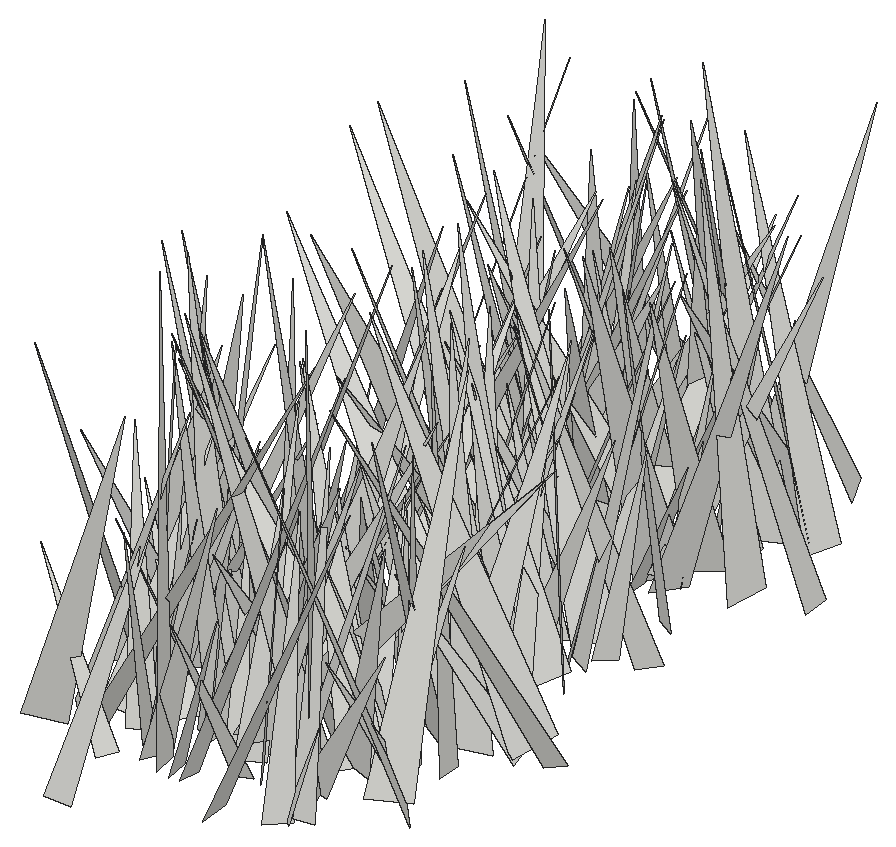
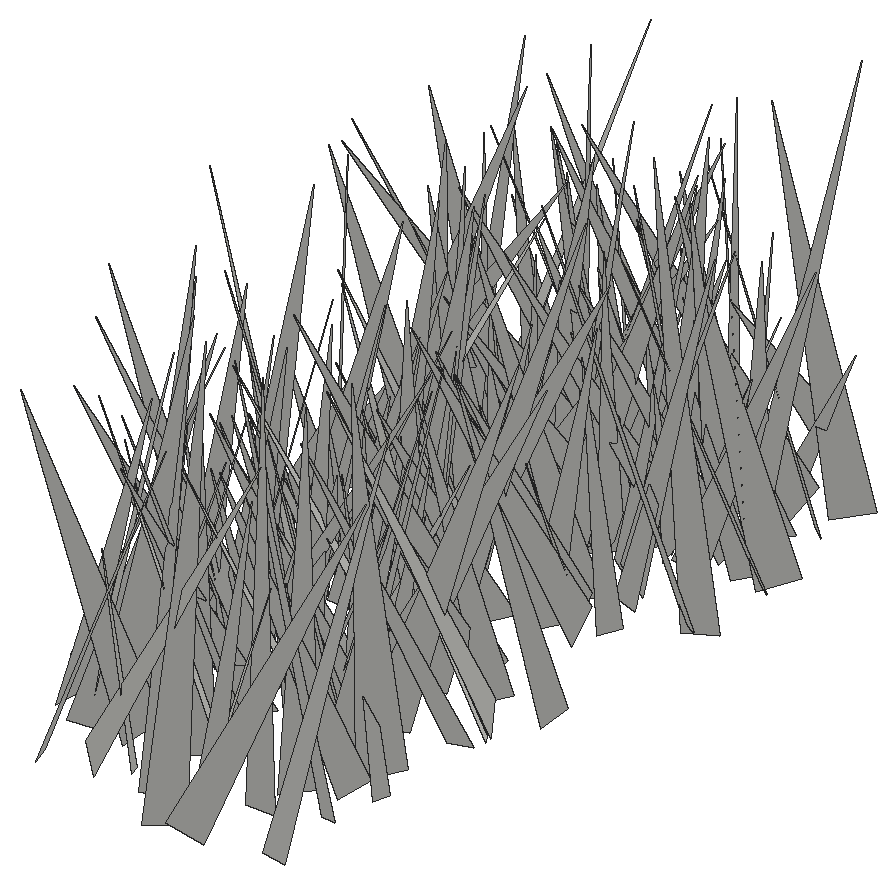
# SketchUp Ruby script. Lengths in inches.
U = 1.inch
M = Sketchup.active_model
def pt(a) = Geom::Point3d.new(a.map { |v| v * U })
def face(e, loops, mat)
  f = e.add_face(loops[0].map { |a| pt(a) })
  loops[1..].each { |l| e.add_face(l.map { |a| pt(a) }).erase! }
  f.material = f.back_material = mat if mat
  f
end
# faces: each face lists its corners as indices into pts; further lists are holes
def faces(e, pts, list, mat = nil) = list.each { |f| face(e, (f[0].is_a?(Array) ? f : [f]).map { |l| l.map { |i| pts[i] } }, mat) }
# xy, xz, yz: faces in a plane at the given z, y or x. An outline is a flat list of corners, or four numbers for a rectangle; further outlines are holes
def ring(l) = l.size == 4 ? [[l[0], l[1]], [l[2], l[1]], [l[2], l[3]], [l[0], l[3]]] : l.each_slice(2).to_a
def flat(e, list, mat, &to3) = list.each { |f| face(e, (f[0].is_a?(Array) ? f : [f]).map { |l| ring(l).map { |u, v| to3.(u, v) } }, mat) }
def xy(e, z, list, mat = nil) = flat(e, list, mat) { |x, y| [x, y, z] }
def xz(e, y, list, mat = nil) = flat(e, list, mat) { |x, z| [x, y, z] }
def yz(e, x, list, mat = nil) = flat(e, list, mat) { |y, z| [x, y, z] }
def lines(e, pts, list) = list.each { |a, b| e.add_line(pt(pts[a]), pt(pts[b])) }
# prism: a flat outline (further loops are holes) pulled along v
def prism(e, loops, v, mat = nil)
  f = face(e, loops, mat); d = Geom::Vector3d.new(v.map { |x| x * U })
  f.pushpull(f.normal.samedirection?(d) ? d.length : -d.length)
end
def box(e, o, s, mat = nil) = prism(e, [[o, [o[0] + s[0], o[1], o[2]], [o[0] + s[0], o[1] + s[1], o[2]], [o[0], o[1] + s[1], o[2]]]], [0, 0, s[2]], mat)
def at(x, y, z, deg = 0) = Geom::Transformation.translation(pt([x, y, z])) * Geom::Transformation.rotation(ORIGIN, Z_AXIS, deg.degrees)
def axes(o, x, y, z) = Geom::Transformation.new([*x, 0, *y, 0, *z, 0, *pt(o).to_a, 1])
def part(name) = M.definitions.add(name)
# library, detail: a bought-in or finely detailed component or shape, given as its bounding box
def library(name, o, s) = part(name).tap { |d| box(d.entities, o, s) }
def detail(e, o, s) = box(e.add_group.entities, o, s)
def put(e, d, t, mat = nil) = e.add_instance(d, t).tap { |i| i.material = mat if mat }
def group(e, t, mat = nil) = e.add_group.tap { |g| g.transformation = t; g.material = mat if mat }.entities
root = M.entities
c1 = part("fur_instance\#9")
p = [[0.8125,0,1.79],[0.67,-0.02,1.48],[0,-0.11,0],[0,0.11,0]]
faces(c1.entities,p,[[0,1,2,3]])
put(root,c1,axes([470.51,80.25,-21.66],[-3.32037,-5.8988,2.51801],[-6.36421,2.67847,-2.11746],[-0.7956,3.19234,6.42939]))
put(root,c1,axes([468.38,101.12,-21.86],[-2.99336,-6.46525,0.18966],[-6.30073,2.9619,1.52434],[1.46161,-0.47255,6.9596]))
put(root,c1,axes([470.64,92.61,-21.66],[-5.74656,4.30747,2.03787],[4.75581,5.38477,2.02895],[0.29923,-2.86007,6.88916]))
put(root,c1,axes([469.65,78.47,-21.66],[1.26749,-5.25605,0.55346],[-5.00773,-1.37633,-1.60227],[-1.68968,0.13629,5.16385]))
put(root,c1,axes([467.07,88.49,-21.86],[6.15775,0.09619,0.89999],[0.03195,-6.20791,0.44493],[-0.90455,0.43558,6.14241]))
put(root,c1,axes([469.07,94.78,-21.86],[-5.99811,4.4385,2.51735],[4.45899,6.44808,-0.74453],[2.48087,-0.8583,7.4245]))
put(root,c1,axes([470.49,72.26,-21.86],[-1.80359,3.13263,0.44398],[3.00697,1.53819,1.36218],[-0.98418,-1.04117,3.34825]))
put(root,c1,axes([468.84,76.53,-21.86],[-3.41876,-7.6362,0.72671],[-7.48826,3.49493,1.49637],[1.66304,0.03883,8.23167]))
put(root,c1,axes([466.91,77.29,-21.86],[5.22316,-4.20753,1.34718],[-4.41725,-5.01042,1.47756],[-0.07792,1.998,6.54228]))
put(root,c1,axes([466.87,81.31,-21.86],[0.15208,-7.64456,1.76209],[-7.47072,0.39677,2.36609],[2.3943,1.72356,7.27077]))
put(root,c1,axes([468.41,89.93,-21.66],[6.47169,4.71895,0.84374],[4.29058,-6.33416,2.51645],[-2.13805,1.57262,7.60387]))
put(root,c1,axes([467.27,77.71,-21.86],[3.93505,4.96293,0.50565],[4.97977,-3.8695,-0.7745],[0.29702,-0.87596,6.28613]))
put(root,c1,axes([469.98,81.29,-21.86],[-1.24841,-4.57565,0.91997],[-4.66472,1.19209,-0.401],[-0.15278,0.99186,4.72592]))
put(root,c1,axes([472.93,89.31,-21.86],[-4.85114,5.94494,0.47809],[5.69058,4.42924,2.66526],[-1.78556,-2.03568,7.19529]))
put(root,c1,axes([471.02,75.84,-21.86],[-2.26305,3.25436,0.20739],[3.19812,2.16563,0.91504],[-0.63708,-0.68879,3.8568]))
put(root,c1,axes([473.08,76.92,-21.86],[-7.866,-1.33504,0.19154],[-1.32695,7.45779,-2.51268],[-0.24134,2.50839,7.5725]))
put(root,c1,axes([468.86,74.78,-21.86],[-1.32926,4.80497,0.97182],[4.66035,1.55098,-1.29408],[1.52094,-0.553,4.81456]))
put(root,c1,axes([470.34,74.24,-21.86],[-1.55203,4.86816,1.43833],[5.0761,1.479,0.47157],[-0.03172,-1.51332,5.08777]))
put(root,c1,axes([467.65,72.6,-21.66],[4.01839,-5.64573,1.18023],[-5.73753,-3.76564,1.52164],[0.58986,1.83314,6.76065]))
put(root,c1,axes([470.63,75.46,-21.86],[-7.01527,0.64484,2.20419],[0.06996,7.14138,-1.86657],[2.29551,1.75305,6.79307]))
put(root,c1,axes([470.91,77.6875,-21.86],[-4.6642,0.46344,0.8289],[0.1067,4.38406,-1.85075],[0.94364,1.79496,4.30631]))
put(root,c1,axes([471.59,101.64,-21.86],[1.60402,-6.13136,0.73735],[-5.58582,-1.76536,-2.52831],[-2.63361,0.00991,5.81155]))
put(root,c1,axes([468.12,95.96,-21.86],[5.21952,0.68023,0.61562],[0.83808,-4.98198,-1.60081],[-0.37326,-1.674,5.01433]))
put(root,c1,axes([467.94,90.85,-21.86],[3.62695,2.69385,0.06353],[2.59465,-3.4627,-1.30122],[0.7271,-1.08099,4.32648]))
put(root,c1,axes([467.18,81.49,-21.66],[5.13352,5.29295,1.04527],[5.31008,-4.70157,-2.27141],[0.95446,-2.31104,7.01492]))
put(root,c1,axes([468.11,73.8125,-21.86],[4.67492,4.49227,1.13099],[4.6277,-4.45606,-1.42912],[0.20972,-1.8104,6.324]))
put(root,c1,axes([468.34,91.6875,-21.86],[1.18506,6.07091,0.5983],[5.8889,-0.9794,-1.72625],[1.5921,-0.89616,5.93973]))
put(root,c1,axes([469.21,82.99,-21.86],[4.35751,-1.25814,0.68683],[-1.21703,-4.4086,-0.35441],[-0.75729,-0.15444,4.52164]))
put(root,c1,axes([473.0625,91.98,-21.66],[-7.26619,-2.16018,0.91047],[-2.32448,7.02333,-1.88745],[0.30351,2.07347,7.34176]))
put(root,c1,axes([471.36,76.4375,-21.86],[-2.85386,-2.94003,0.13695],[-2.93623,2.85714,0.14971],[0.2028,-0.00613,4.09462]))
put(root,c1,axes([471.38,77.2,-21.86],[-7.46216,1.5868,2.36089],[1.65538,7.81249,-0.01867],[2.31332,-0.47194,7.62898]))
put(root,c1,axes([471.58,93.05,-21.86],[-6.2182,-2.45212,1.53392],[-2.39925,6.40419,0.51167],[1.61537,0.0727,6.66461]))
put(root,c1,axes([471.03,82.51,-21.66],[1.74005,3.73475,0.21366],[3.48509,-1.70407,1.40429],[-1.35946,0.41179,3.87351]))
put(root,c1,axes([470.57,95.25,-21.86],[3.73723,-3.51523,0.8829],[-3.22394,-3.80362,-1.49732],[-1.65607,-0.52811,4.90732]))
put(root,c1,axes([471.1,68.95,-21.86],[-4.90566,2.32822,0.51514],[1.6552,4.17303,-3.098],[1.71648,2.62995,4.45965]))
put(root,c1,axes([470.23,87.96,-21.86],[5.42222,1.22065,1.50489],[0.3801,-5.05507,2.73075],[-1.90005,2.47215,4.84081]))
put(root,c1,axes([468.04,77.6,-21.86],[0.54416,-5.67013,1.84078],[-5.27926,0.40028,2.79359],[2.76917,1.87733,4.9641]))
put(root,c1,axes([470.67,74.41,-21.86],[-4.89725,-3.9807,3.26033],[-4.56553,5.43754,-0.21877],[2.37312,2.24631,6.30723]))
put(root,c1,axes([470.1,83.29,-21.86],[7.02675,2.35333,1.41841],[1.60681,-6.67867,3.12071],[-2.22895,2.60433,6.72121]))
put(root,c1,axes([471.99,75.27,-21.86],[4.59054,6.55576,1.84003],[6.00661,-4.94402,2.62946],[-3.20693,0.124,7.5589]))
put(root,c1,axes([471.59,89.53,-21.86],[6.1806,-4.85252,1.92283],[-3.89661,-6.27237,-3.30423],[-3.47285,-1.59827,7.12944]))
put(root,c1,axes([471.51,79.5625,-21.86],[-3.91198,-5.41617,1.52932],[-5.50053,4.07361,0.35664],[1.19076,1.02376,6.67167]))
put(root,c1,axes([470.56,74.21,-21.86],[2.84043,2.51238,0.82611],[2.52394,-2.93724,0.2547],[-0.79009,-0.35083,3.78354]))
put(root,c1,axes([468.93,96.34,-21.66],[5.6454,-1.61471,0.55375],[-1.70236,-5.46688,1.41409],[-0.12614,1.5134,5.69896]))
put(root,c1,axes([470.64,74.18,-21.86],[4.23217,0.79223,1.75299],[1.35483,-4.23497,-1.35698],[-1.36567,-1.74623,4.08626]))
put(root,c1,axes([468.37,98.36,-21.66],[5.01746,5.30698,2.27397],[5.71554,-4.13917,-2.95123],[0.81705,-3.63499,6.68051]))
put(root,c1,axes([470.44,97.27,-21.86],[5.51508,-3.1001,1.56666],[-3.03836,-5.73026,-0.64316],[-1.68328,0.18611,6.29389]))
put(root,c1,axes([469.2,76.88,-21.66],[5.44463,0.12063,0.24069],[0.04962,-5.23956,1.50366],[-0.26462,1.49964,5.23426]))
put(root,c1,axes([470.77,82.32,-21.86],[5.48783,2.36239,1.1528],[1.72376,-5.24883,2.55038],[-1.98455,1.97355,5.40302]))
put(root,c1,axes([472.52,72.66,-21.66],[-7.45834,-2.27512,2.73301],[-2.96816,7.48025,-1.87304],[1.95846,2.67246,7.56933]))
put(root,c1,axes([472.49,75.58,-21.86],[-6.61174,-0.50833,1.66504],[-0.62205,6.79727,-0.39495],[1.62598,0.53342,6.61948]))
put(root,c1,axes([470.8125,83.7,-21.86],[-3.2571,5.60614,0.8435],[5.30317,3.35677,-1.83235],[2.00417,0.22864,6.21933]))
put(root,c1,axes([469.28,88.66,-21.86],[3.19208,-3.97574,0.46961],[-3.91795,-2.97897,1.41133],[0.82265,1.2392,4.89939]))
put(root,c1,axes([472.45,78.92,-21.66],[-6.55431,0.09701,1.7896],[-0.34688,6.588,-1.62754],[1.75834,1.66126,6.34976]))
put(root,c1,axes([472.17,82.44,-21.86],[-0.83956,4.61048,2.28414],[5.1209,0.52371,0.82514],[-0.50027,-2.37653,4.61309]))
put(root,c1,axes([472.4,95.2,-21.86],[-4.41173,-1.92667,0.46008],[-1.77307,4.34177,1.17998],[0.88316,-0.90777,4.66723]))
put(root,c1,axes([470.45,99.21,-21.66],[-1.45623,-6.82166,1.9418],[-6.84757,1.86878,1.42991],[1.84835,1.54881,6.82723]))
put(root,c1,axes([469.75,76.44,-21.86],[3.43659,4.37627,1.35344],[4.55407,-3.08156,-1.59944],[0.49399,-2.03617,5.32951]))
put(root,c1,axes([475.37,83.7,-21.86],[-5.71693,5.39586,0.3581],[5.20349,5.34707,2.50186],[-1.47216,-2.05434,7.45247]))
put(root,c1,axes([472.47,91.63,-21.86],[-5.1029,2.41175,1.4356],[2.37658,5.2976,-0.4521],[1.4931,-0.1897,5.62599]))
put(root,c1,axes([472.86,98.9375,-21.86],[-3.26871,-2.2439,0.63682],[-2.29753,3.28654,-0.21245],[0.40248,0.53729,3.95909]))
put(root,c1,axes([471.55,76.61,-21.86],[6.78257,3.66457,1.14232],[2.83952,-6.35069,3.51329],[-2.58286,2.6414,6.86216]))
put(root,c1,axes([473.46,80.1,-21.66],[-0.04463,-6.97717,1.39975],[-6.92736,-0.27772,-1.60522],[-1.62845,1.37265,6.79015]))
put(root,c1,axes([471.07,94.03,-21.86],[3.65147,4.43575,1.22236],[4.5601,-3.69672,-0.20725],[-0.61278,-1.07778,5.74161]))
put(root,c1,axes([472.53,99.3,-21.86],[-1.33118,-5.02308,1.66852],[-5.29255,1.28443,-0.35575],[0.06525,1.70478,5.18429]))
put(root,c1,axes([472.21,82.57,-21.66],[-4.0426,1.99311,1.15136],[1.52694,4.06338,-1.67276],[1.72237,1.07573,4.18533]))
put(root,c1,axes([471.67,94.47,-21.66],[4.6203,4.92142,0.32663],[4.69042,-4.52255,1.79463],[-1.52544,1.00021,6.50745]))
put(root,c1,axes([469.33,72.95,-21.66],[7.73901,0.54751,0.09462],[0.50511,-7.48314,1.98706],[-0.23147,1.9758,7.49957]))
put(root,c1,axes([473,89.42,-21.86],[-0.62514,-3.66803,1.11265],[-3.82799,0.53943,-0.37244],[-0.19721,1.15663,3.70223]))
put(root,c1,axes([470.14,87.85,-21.66],[7.35163,-0.33714,0.71191],[-0.54127,-7.01692,2.26646],[-0.57229,2.30568,7.00167]))
put(root,c1,axes([472.29,84.82,-21.66],[-2.9389,4.8588,0.20427],[4.55933,2.83593,-1.85926],[1.6918,0.79774,5.36547]))
put(root,c1,axes([474.28,89.21,-21.86],[-2.77092,-3.22119,0.17285],[-3.17409,2.68192,-0.90354],[-0.57541,0.71776,4.15182]))
put(root,c1,axes([473.98,79.47,-21.86],[-7.67624,-2.38765,2.18106],[-2.53698,7.93,-0.24775],[2.0054,0.89261,8.03519]))
put(root,c1,axes([473.28,75.37,-21.86],[-0.33834,3.74046,0.53618],[3.75079,0.26714,0.50319],[-0.45836,-0.57497,3.72187]))
put(root,c1,axes([474.47,87.67,-21.66],[0.43766,-5.35462,0.13989],[-4.92597,-0.45748,-2.09965],[-2.10387,-0.04276,4.94519]))
put(root,c1,axes([472.75,79.39,-21.86],[3.27584,-2.78093,0.2499],[-2.38988,-2.99185,-1.96583],[-1.44378,-1.35736,3.82103]))
put(root,c1,axes([471.39,76.43,-21.86],[3.86855,-0.79855,0.19754],[-0.81455,-3.85123,0.38332],[-0.11496,0.41562,3.93147]))
put(root,c1,axes([472,95.17,-21.86],[5.42096,2.25752,1.64956],[2.38588,-5.61122,-0.16143],[-1.45775,-0.7887,5.87002]))
put(root,c1,axes([476.5,78.19,-21.66],[-6.39943,2.86094,0.01202],[2.71801,6.07041,2.2137],[-0.89308,-2.0256,6.65111]))
put(root,c1,axes([473.33,93.72,-21.86],[0.82489,5.68831,1.342],[5.81529,-0.93413,0.38496],[-0.58339,-1.2684,5.73491]))
put(root,c1,axes([471.18,81.78,-21.86],[2.35297,-5.60644,2.50548],[-6.03434,-1.6135,2.05656],[1.13856,3.03489,5.72182]))
put(root,c1,axes([471.32,92.89,-21.66],[6.28882,0.29269,0.74734],[0.08478,-6.11246,1.68051],[-0.79813,1.65699,6.06719]))
put(root,c1,axes([471.73,73.21,-21.86],[5.0608,-1.8582,0.79428],[-1.91101,-5.09708,0.2516],[-0.65714,0.51221,5.38529]))
put(root,c1,axes([475.91,77.33,-21.66],[-4.08084,-6.31933,0.93728],[-6.28934,3.77891,-1.90517],[-1.12095,1.80323,7.27719]))
put(root,c1,axes([472,81.39,-21.86],[4.40688,2.08061,0.00975],[2.02682,-4.29803,1.08102],[-0.47012,0.97349,4.75194]))
put(root,c1,axes([476.33,93.375,-21.86],[-7.00038,0.48524,0.02911],[0.47648,6.76613,1.79834],[-0.09628,-1.796,6.78283]))
put(root,c1,axes([475.12,93.96,-21.86],[-4.76571,-0.2474,0.30777],[-0.30187,4.68534,-0.90794],[0.25457,0.92426,4.68496]))
put(root,c1,axes([470.7,94.47,-21.66],[2.62599,-5.06265,0.78885],[-4.77605,-2.09765,2.43674],[1.85526,1.76578,5.15641]))
put(root,c1,axes([474.54,74.5,-21.66],[-5.37291,2.30629,0.61766],[1.96946,5.14098,-2.06404],[1.34972,1.6793,5.47055]))
put(root,c1,axes([475.92,76.06,-21.86],[-7.9003,-1.05971,0.99848],[-1.05239,7.96314,0.1246],[1.0062,0.00826,7.97008]))
put(root,c1,axes([472.47,101.57,-21.86],[7.22069,-3.00234,1.05262],[-2.62839,-7.10035,-2.22196],[-1.79266,-1.6827,7.49769]))
put(root,c1,axes([476.98,99.72,-21.86],[-4.9499,-5.12629,0.49866],[-4.98162,4.58947,-2.26921],[-1.30806,1.92014,6.75508]))
put(root,c1,axes([473.76,88.27,-21.86],[5.15692,6.28398,0.1894],[5.87834,-4.90651,2.73667],[-2.22922,1.59869,7.6546]))
put(root,c1,axes([474.41,83.51,-21.86],[-3.76395,0.54517,1.33918],[0.93594,3.7652,1.09781],[1.1021,-1.33566,3.64133]))
put(root,c1,axes([476.24,97.53,-21.86],[-6.46812,-3.13785,1.21731],[-3.3431,6.29489,-1.53709],[0.38946,1.92167,7.02282]))
put(root,c1,axes([472.86,72.83,-21.86],[3.7872,-0.0255,0.26622],[0.02172,-3.73751,-0.66706],[-0.26655,-0.66693,3.72808]))
put(root,c1,axes([472.92,87.74,-21.86],[4.18181,1.0835,0.53294],[1.13424,-4.18373,-0.39425],[-0.41412,-0.51766,4.30187]))
put(root,c1,axes([472.74,94.25,-21.86],[0.16634,-6.6201,0.01552],[-6.42128,-0.15757,1.61124],[1.61035,0.05552,6.42319]))
put(root,c1,axes([470.91,98.16,-21.86],[4.45492,4.83666,0.95124],[4.56601,-3.56591,-3.25273],[1.85733,-2.83468,5.71483]))
put(root,c1,axes([474.77,73.84,-21.86],[0.53786,-3.60504,0.14249],[-3.55289,-0.5543,-0.6129],[-0.62738,0.04841,3.59304]))
put(root,c1,axes([472.51,78.08,-21.66],[5.53562,0.75174,0.06867],[0.66774,-5.11345,2.14935],[-0.35205,2.12143,5.1564]))
put(root,c1,axes([472.46,87.64,-21.86],[6.04949,2.12455,0.78775],[2.22415,-5.99674,-0.90711],[-0.43293,-1.1207,6.34722]))
put(root,c1,axes([472.77,82.79,-21.86],[5.43533,-0.93824,0.08866],[-0.80913,-4.91198,-2.3767],[-0.48317,-2.32876,4.97739]))
put(root,c1,axes([474.22,83.47,-21.66],[-2.58943,-3.13022,0.07236],[-2.65217,2.2427,2.10831],[1.66419,-1.2964,3.47253]))
put(root,c1,axes([473.61,72.55,-21.66],[6.82922,2.21825,1.16198],[1.82522,-6.72015,2.10172],[-1.71447,1.68168,6.86597]))
put(root,c1,axes([474.5625,88.73,-21.86],[0.52075,4.40411,1.27547],[4.58416,-0.47433,-0.2338],[0.09203,-1.29345,4.42863]))
put(root,c1,axes([472,78.8,-21.66],[1.01842,-6.5564,0.3467],[-5.92672,-0.76709,2.90332],[2.82498,0.75429,5.9661]))
put(root,c1,axes([475.28,85.61,-21.86],[3.99343,-3.31881,2.86458],[-3.84361,-4.5142,0.12826],[-2.10878,1.94301,5.19091]))
put(root,c1,axes([474.54,95.67,-21.86],[3.11347,-5.57932,0.56956],[-5.54553,-3.1599,-0.63956],[-0.83685,0.18197,6.35716]))
put(root,c1,axes([474.7,88.55,-21.86],[5.01646,-0.03484,2.02413],[0.79085,-4.94522,-2.0451],[-1.86357,-2.19241,4.58078]))
put(root,c1,axes([475.57,91.15,-21.86],[-6.08575,-1.31512,1.93305],[-0.80976,6.24223,1.69745],[2.19329,-1.34444,5.99037]))
put(root,c1,axes([472.75,78.29,-21.86],[6.6655,-1.52718,0.22941],[-1.49066,-6.62814,-0.81212],[-0.40351,-0.74118,6.78982]))
put(root,c1,axes([476.13,83.74,-21.86],[-6.8866,-1.44069,2.04712],[-1.4724,7.17733,0.09795],[2.02444,0.3193,7.035]))
put(root,c1,axes([475.52,78.89,-21.86],[-3.08367,2.72536,1.78242],[3.08151,3.23588,0.38343],[1.05304,-1.48834,4.09751]))
put(root,c1,axes([474.39,89.83,-21.66],[4.68389,2.5085,0.46697],[2.25732,-4.52881,1.68637],[-1.1896,1.28326,5.03861]))
put(root,c1,axes([474.47,75.05,-21.66],[4.97283,-0.90694,1.68915],[-1.45035,-4.85051,1.66547],[-1.25389,2.01364,4.77261]))
put(root,c1,axes([476.92,83.34,-21.86],[-1.73257,6.85044,2.42635],[7.20837,1.30251,1.46979],[-0.92468,-2.68187,6.91158]))
put(root,c1,axes([477.31,88.67,-21.86],[-5.50457,-1.9976,0.13924],[-1.94432,5.42927,1.02602],[0.47897,-0.91798,5.76524]))
put(root,c1,axes([474.51,97.46,-21.86],[4.37125,-4.19897,0.80164],[-4.19734,-4.43318,-0.33332],[-0.81017,0.31203,6.05212]))
put(root,c1,axes([474.55,94.13,-21.86],[-2.22642,5.28944,0.76409],[4.89566,2.35054,-2.00661],[2.14349,0.12554,5.37668]))
put(root,c1,axes([473.91,100.625,-21.66],[-3.7888,-7.35051,1.42507],[-6.56657,4.02946,3.32556],[3.59735,-0.38635,7.57137]))
put(root,c1,axes([475.1,74.39,-21.86],[4.36466,2.86173,1.95624],[3.18404,-4.55325,-0.44325],[-1.3705,-1.46462,5.20032]))
put(root,c1,axes([477.3,76.73,-21.86],[-5.2406,4.407,1.34408],[4.57378,5.22157,0.71269],[0.55566,-1.41624,6.81011]))
put(root,c1,axes([479.58,82.87,-21.86],[-7.14593,-4.06809,0.00282],[-3.91681,6.87864,-2.22635],[-1.09909,1.93614,7.91562]))
put(root,c1,axes([473.56,85.1,-21.66],[2.80072,3.68056,0.20092],[3.50306,-2.57922,-1.58339],[1.14693,-1.10998,4.34551]))
put(root,c1,axes([477.17,84.43,-21.66],[-0.80473,7.1427,2.6366],[7.51279,0.31449,1.44102],[-1.23607,-2.73867,7.04196]))
put(root,c1,axes([473.32,97.42,-21.66],[5.31801,3.62577,0.57345],[3.65614,-5.14142,-1.39812],[0.32822,-1.47507,6.28273]))
put(root,c1,axes([476.07,80.88,-21.86],[-0.63245,-3.70623,0.66325],[-3.76509,0.62047,-0.12308],[-0.01169,0.67448,3.75779]))
put(root,c1,axes([476.92,86.97,-21.86],[0.57769,-3.84784,2.16026],[-4.16363,-1.197,-1.01866],[-1.46176,1.88882,3.75525]))
put(root,c1,axes([473.63,75.71,-21.66],[5.89458,-2.32049,1.52507],[-2.76984,-5.16651,2.8446],[-0.1962,3.22166,5.6603]))
put(root,c1,axes([476.33,93.875,-21.86],[-5.52668,-3.91053,1.22579],[-3.5737,5.60606,1.77193],[2.00587,-0.78663,6.53427]))
put(root,c1,axes([478.09,87.77,-21.86],[-6.89397,4.20656,1.53795],[4.42912,6.82252,1.19307],[0.66584,-1.82904,7.9874]))
put(root,c1,axes([475.08,92.88,-21.86],[4.10361,0.18993,0.89205],[0.09258,-4.17709,0.46346],[-0.90734,0.43277,4.08178]))
put(root,c1,axes([476.49,89.52,-21.86],[-3.67064,-4.64361,1.03864],[-4.58105,3.8034,0.81465],[1.28682,0.29416,5.86285]))
put(root,c1,axes([478.44,95.3,-21.86],[-5.31837,-1.43549,0.4315],[-1.49067,5.23198,-0.96754],[0.15722,1.04767,5.42306]))
put(root,c1,axes([478.45,84.89,-21.86],[-6.01632,2.22797,0.81671],[2.32649,5.97644,0.83455],[0.46722,-1.07014,6.36109]))
put(root,c1,axes([475.38,99.45,-21.86],[3.34183,1.38887,0.77255],[1.56239,-3.2005,-1.00466],[-0.29109,-1.23347,3.4767]))
put(root,c1,axes([475.88,84.34,-21.86],[2.91229,5.1803,0.24137],[5.15397,-2.92189,0.52374],[-0.57474,0.04729,5.91968]))
put(root,c1,axes([478.4,96.26,-21.86],[-0.9931,7.68396,2.84346],[8.04191,0.36629,1.81887],[-1.56723,-2.98953,7.53135]))
put(root,c1,axes([474.87,82.41,-21.86],[5.42276,2.60915,0.23648],[2.58182,-5.41452,0.53583],[-0.44475,0.3811,5.9939]))
put(root,c1,axes([477.55,74.06,-21.86],[-6.98093,-2.98191,2.95578],[-3.56155,7.24267,-1.10492],[2.22346,2.23913,7.51028]))
put(root,c1,axes([477.75,78.23,-21.86],[-3.47043,-1.20582,0.35373],[-1.16309,3.47557,0.43669],[0.47575,-0.29913,3.64791]))
put(root,c1,axes([477.1,77.42,-21.86],[-1.60634,4.05647,0.77587],[4.09581,1.67158,-0.25963],[0.53033,-0.623,4.35521]))
put(root,c1,axes([477.51,72.15,-21.86],[-4.49774,2.41965,1.22715],[2.26445,4.65664,-0.88215],[1.49428,0.22634,5.03052]))
put(root,c1,axes([476.15,95.42,-21.86],[-0.58036,-3.55618,1.37675],[-3.59236,0.97706,1.00942],[1.27936,1.13031,3.45894]))
put(root,c1,axes([476.98,79.88,-21.86],[-5.03968,3.97301,2.20808],[3.85689,5.48236,-1.06156],[2.40517,-0.46656,6.329]))
put(root,c1,axes([478.34,100.55,-21.86],[-5.06216,-2.56794,0.53616],[-2.44101,5.03776,1.08155],[0.96086,-0.73072,5.57226]))
put(root,c1,axes([478.31,83.34,-21.66],[-4.48023,1.71415,0.10108],[1.53614,4.12726,-1.90446],[0.76734,1.74596,4.4027]))
put(root,c1,axes([478.21,72.52,-21.66],[1.19098,5.93826,0.851],[5.76454,-1.37303,1.51343],[-1.66049,-0.50738,5.86438]))
put(root,c1,axes([477.74,78.15,-21.86],[-3.90689,0.46662,1.17538],[0.26281,4.03296,-0.72751],[1.23701,0.61693,3.86682]))
put(root,c1,axes([477.62,95.5625,-21.86],[3.95748,1.9361,2.48086],[2.44941,-4.39763,-0.47534],[-1.97573,-1.57388,4.37997]))
put(root,c1,axes([476.94,89.0625,-21.86],[0.96438,4.41888,0.40988],[4.43511,-0.94495,-0.24768],[0.15571,-0.45288,4.5161]))
put(root,c1,axes([476.72,97.36,-21.86],[6.67924,-1.26552,2.75336],[-2.18749,-6.62541,2.26131],[-2.097,2.88046,6.41095]))
put(root,c1,axes([480.39,87.4375,-21.86],[-1.48445,-5.73193,2.26963],[-5.6541,0.33538,-2.85107],[-2.45713,2.69116,5.18942]))
put(root,c1,axes([477.03,92.22,-21.86],[5.51708,-5.76072,0.82028],[-5.55442,-5.55067,-1.6234],[-1.73412,-0.54876,7.80952]))
put(root,c1,axes([479.93,96.84,-21.86],[-6.93734,1.12272,0.61983],[1.08478,6.95591,-0.45824],[0.68406,0.3553,7.01265]))
put(root,c1,axes([478.99,97.34,-21.86],[-5.18557,-4.32883,1.54546],[-4.49087,5.26797,-0.31293],[0.97941,1.23577,6.74766]))
put(root,c1,axes([475.5,71.46,-21.86],[6.47298,0.85818,0.33872],[0.84258,-6.4766,0.30739],[-0.37587,0.26066,6.52238]))
put(root,c1,axes([477.36,94.42,-21.86],[3.56693,3.32971,1.1246],[3.34181,-3.70943,0.38354],[-1.08812,-0.47732,4.86445]))
put(root,c1,axes([478.24,85.99,-21.86],[3.78632,3.0497,0.88341],[2.42458,-3.66486,2.25998],[-2.05,1.29824,4.30457]))
put(root,c1,axes([477.84,82.35,-21.66],[-4.12038,-2.11418,1.50488],[-1.47976,4.23386,1.89649],[2.13184,-1.14743,4.225]))
put(root,c1,axes([479.15,89.82,-21.86],[-3.42512,-4.29344,1.99666],[-4.721,3.28594,-1.03273],[0.36395,2.21827,5.39431]))
put(root,c1,axes([476.64,86.25,-21.86],[3.70527,-2.55389,0.75103],[-2.66189,-3.54115,1.0909],[0.02774,1.32414,4.36593]))
put(root,c1,axes([477.45,92.3,-21.86],[1.48907,3.83094,1.46531],[4.09712,-1.31638,-0.722],[0.19182,-1.62223,4.04625]))
put(root,c1,axes([477.43,72.625,-21.86],[4.30738,5.01035,0.65824],[4.94004,-4.35705,0.83813],[-1.06435,0.05398,6.55397]))
put(root,c1,axes([473.18,79.28,-21.86],[5.03462,6.0848,0.40692],[5.07887,-3.8915,-4.64748],[3.37572,-3.22012,6.38538]))
put(root,c1,axes([473.56,76.7,-21.66],[6.0984,-4.54505,0.22334],[-3.82324,-4.91501,4.37303],[2.46783,3.61705,6.22291]))
put(root,c1,axes([479.375,79.7,-21.86],[-0.74799,6.94474,2.29097],[7.27165,0.46217,0.97314],[-0.77532,-2.36525,6.91678]))
put(root,c1,axes([478.35,98.12,-21.86],[4.64507,-4.79979,0.2726],[-4.36308,-4.36804,-2.56373],[-2.01887,-1.6035,6.16782]))
put(root,c1,axes([477.97,93.55,-21.86],[3.11864,-5.68803,0.55795],[-5.6529,-3.16353,-0.65398],[-0.84244,0.17118,6.45383]))
put(root,c1,axes([479.6875,78.14,-21.86],[-6.31895,-1.30533,1.91515],[-1.71826,6.37081,-1.32708],[1.5554,1.73484,6.31441]))
put(root,c1,axes([478.51,86.23,-21.86],[3.93079,5.90323,1.06815],[5.73682,-4.07234,1.39466],[-1.7544,-0.09002,6.95371]))
put(root,c1,axes([481.02,80.81,-21.66],[-7.69272,2.37823,1.5322],[2.71051,7.46743,2.01798],[0.8104,-2.40066,7.79498]))
put(root,c1,axes([480.29,75.3,-21.86],[-5.65228,-5.31186,0.60473],[-5.29476,5.68375,0.43618],[0.73959,0.09466,7.74428]))
put(root,c1,axes([476.87,91.12,-21.86],[6.67299,1.88656,0.54903],[1.75109,-6.59185,1.3677],[-0.89119,1.17381,6.79833]))
put(root,c1,axes([482.32,80.28,-21.66],[-2.35699,-6.63901,0.53799],[-6.01099,1.87426,-3.2057],[-2.86948,1.52709,6.27339]))
put(root,c1,axes([476.08,89.51,-21.66],[7.20484,3.15988,1.15153],[3.35999,-6.88107,-2.14053],[-0.14588,-2.42624,7.57051]))
put(root,c1,axes([482.07,93.8,-21.86],[-7.1325,-1.97369,0.04131],[-1.9512,7.0246,-1.27181],[-0.29997,1.23662,7.29044]))
put(root,c1,axes([478.71,85.13,-21.86],[-4.90081,-4.60842,2.76686],[-4.75517,5.4628,0.67611],[2.50627,1.35324,6.69315]))
put(root,c1,axes([477.34,92.03,-21.66],[5.30796,-1.91017,1.71118],[-2.50762,-4.68997,2.54311],[-0.53734,3.01775,5.03546]))
put(root,c1,axes([477.13,76.51,-21.86],[0.27487,-5.90315,0.86813],[-5.62576,0.03312,2.00651],[1.98787,0.91,5.55848]))
put(root,c1,axes([478.9,77.29,-21.86],[5.38301,1.51294,2.42188],[1.75431,-5.82988,-0.25732],[-2.2532,-0.92457,5.58566]))
put(root,c1,axes([478.16,77.03,-21.86],[1.17442,4.10835,0.87727],[4.16659,-1.02282,-0.78793],[0.5364,-1.0501,4.19964]))
put(root,c1,axes([478.27,79.42,-21.86],[-2.59583,-7.17613,0.91864],[-6.91744,2.74775,1.9178],[2.11891,0.17907,7.38629]))
put(root,c1,axes([477.03,74.6,-21.86],[1.43751,-4.12245,0.23292],[-3.7226,-1.18725,1.96162],[1.78636,0.84328,3.90039]))
put(root,c1,axes([479.99,92.91,-21.86],[-7.15931,0.95304,2.49675],[1.12982,7.54938,0.35801],[2.42189,-0.70454,7.21359]))
put(root,c1,axes([479.4,76.46,-21.86],[-3.37323,-1.69913,0.74168],[-1.13548,3.11072,1.96213],[1.46554,-1.50074,3.22735]))
put(root,c1,axes([480.77,80.45,-21.86],[-4.09373,-0.36711,0.23804],[-0.24891,3.79616,1.57392],[0.35983,-1.55061,3.79686]))
put(root,c1,axes([477.73,91.79,-21.86],[6.84778,-1.68967,1.39359],[-1.92956,-6.81846,1.21431],[-1.03628,1.53061,6.94784]))
put(root,c1,axes([479.01,86.94,-21.86],[3.29573,-2.04708,1.27302],[-2.29025,-3.33183,0.57152],[-0.75223,1.17531,3.83742]))
put(root,c1,axes([479.56,75.23,-21.66],[-4.86903,5.31705,1.90275],[5.12727,5.21523,-1.45307],[2.36698,-0.35954,7.06166]))
put(root,c1,axes([478.61,80.03,-21.86],[-2.09917,6.50868,2.06271],[6.47308,2.58358,-1.56477],[2.17184,-1.40938,6.65739]))
